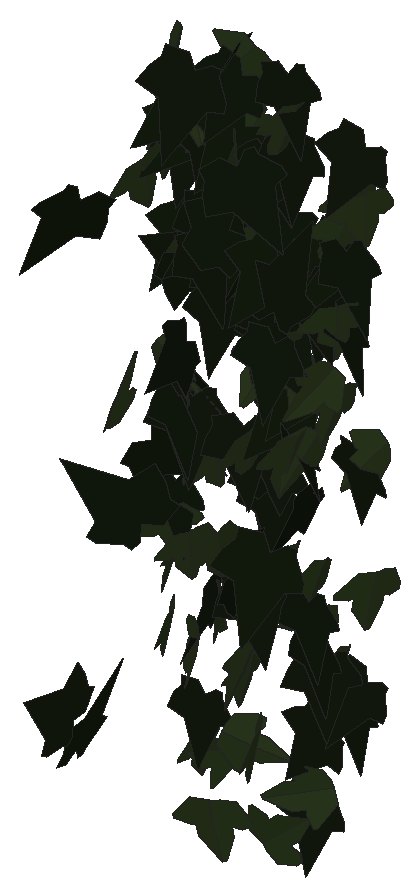
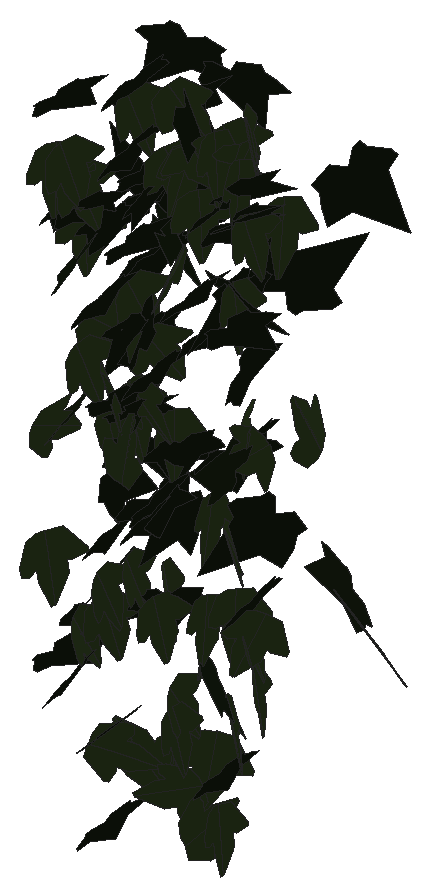
# SketchUp Ruby script. Lengths in inches.
U = 1.inch
M = Sketchup.active_model
def pt(a) = Geom::Point3d.new(a.map { |v| v * U })
def face(e, loops, mat)
  f = e.add_face(loops[0].map { |a| pt(a) })
  loops[1..].each { |l| e.add_face(l.map { |a| pt(a) }).erase! }
  f.material = f.back_material = mat if mat
  f
end
# faces: each face lists its corners as indices into pts; further lists are holes
def faces(e, pts, list, mat = nil) = list.each { |f| face(e, (f[0].is_a?(Array) ? f : [f]).map { |l| l.map { |i| pts[i] } }, mat) }
# xy, xz, yz: faces in a plane at the given z, y or x. An outline is a flat list of corners, or four numbers for a rectangle; further outlines are holes
def ring(l) = l.size == 4 ? [[l[0], l[1]], [l[2], l[1]], [l[2], l[3]], [l[0], l[3]]] : l.each_slice(2).to_a
def flat(e, list, mat, &to3) = list.each { |f| face(e, (f[0].is_a?(Array) ? f : [f]).map { |l| ring(l).map { |u, v| to3.(u, v) } }, mat) }
def xy(e, z, list, mat = nil) = flat(e, list, mat) { |x, y| [x, y, z] }
def xz(e, y, list, mat = nil) = flat(e, list, mat) { |x, z| [x, y, z] }
def yz(e, x, list, mat = nil) = flat(e, list, mat) { |y, z| [x, y, z] }
def lines(e, pts, list) = list.each { |a, b| e.add_line(pt(pts[a]), pt(pts[b])) }
# prism: a flat outline (further loops are holes) pulled along v
def prism(e, loops, v, mat = nil)
  f = face(e, loops, mat); d = Geom::Vector3d.new(v.map { |x| x * U })
  f.pushpull(f.normal.samedirection?(d) ? d.length : -d.length)
end
def box(e, o, s, mat = nil) = prism(e, [[o, [o[0] + s[0], o[1], o[2]], [o[0] + s[0], o[1] + s[1], o[2]], [o[0], o[1] + s[1], o[2]]]], [0, 0, s[2]], mat)
def at(x, y, z, deg = 0) = Geom::Transformation.translation(pt([x, y, z])) * Geom::Transformation.rotation(ORIGIN, Z_AXIS, deg.degrees)
def axes(o, x, y, z) = Geom::Transformation.new([*x, 0, *y, 0, *z, 0, *pt(o).to_a, 1])
def part(name) = M.definitions.add(name)
# library, detail: a bought-in or finely detailed component or shape, given as its bounding box
def library(name, o, s) = part(name).tap { |d| box(d.entities, o, s) }
def detail(e, o, s) = box(e.add_group.entities, o, s)
def put(e, d, t, mat = nil) = e.add_instance(d, t).tap { |i| i.material = mat if mat }
def group(e, t, mat = nil) = e.add_group.tap { |g| g.transformation = t; g.material = mat if mat }.entities
root = M.entities
M.materials.add("efeu1").color = [18, 25, 13]
M.materials.add("efeu2").color = [43, 57, 29]
c1 = part("ivyleaf_9")
p = [[1.54,2.16,1.25],[1.36,2.04,1.19],[-0.21,0.99,0.68],[-0.71,1.11,0.82],[-0.85,0.86,0.67],[-0.8,0.17,0.21],
  [-0.9,-0.01,0.1],[-0.67,-0.16,-0.02],[-0.08,-0.08,-0.05],[-0.03,-0.6,-0.4],[0.65,-0.88,-0.66],[0.83,-0.6,-0.49],
  [1.29,-0.42,-0.43],[1.8125,-0.07,-0.26],[1.21,0.44,0.15]]
faces(c1.entities,p,[[0,1,2,3,4,5,6,7,8,9,10,11,12,13,14]],"efeu1")
c2 = part("ivyleaf_10")
p = [[0,0.5,-0.03],[-0.0625,2.02,-0.43],[-0.19,2.01,-0.46],[-0.54,1.05,-0.29],[-0.52,0.625,-0.18],[-0.83,0.76,-0.28],
  [-1.16,0.64,-0.33],[-1.15,0.33,-0.24],[-0.77,-0.39,0.02],[-0.3,-0.51,0.16],[0.04,-0.48,0.23],[-0.02,2.01,-0.4375],
  [-0.06,2.01,-0.43],[0.04,-0.49,0.23],[0.67,-0.49,0.14],[1.38,0.36,-0.2],[1.375,0.51,-0.24],[0.81,0.65,-0.19],
  [0.62,0.59,-0.15],[0.6,1.09,-0.28],[0.5,1.23,-0.31]]
faces(c2.entities,p,[[0,1,2,3,4,5,6,7,8,9,10],[11,12,0,13,14,15,16,17,18,19,20]],"efeu2")
put(root,c1,axes([543.49,116.36,261.25],[0.16021,0.13331,1.3584],[-1.36181,-0.07688,0.16816],[0.0923,-1.36566,0.12313]))
put(root,c1,axes([539.99,117.03,249.64],[-0.79435,1.04419,-0.28104],[-0.1795,0.21655,1.31195],[1.06635,0.8143,0.01149]))
put(root,c1,axes([538.28,118.64,249.51],[-0.68634,0.81521,0.76926],[-0.53972,0.5502,-1.06461],[-0.98237,-0.87185,0.04745]))
put(root,c1,axes([536.61,121.2,270.97],[-0.0962,0.58477,-1.146],[0.09794,-1.14254,-0.59122],[-1.28284,-0.13108,0.0408]))
put(root,c2,axes([545.42,121.33,250.04],[0.48425,-1.06011,-0.21104],[-0.05067,0.20873,-1.16479],[1.07972,0.48525,0.03998]))
put(root,c1,axes([543.87,122.2,274.54],[-0.28215,-0.65621,-1.04476],[0.69961,0.79766,-0.68994],[1.01621,-0.73135,0.18491]))
put(root,c1,axes([544.65,123.08,257.12],[-0.95258,-0.80439,-0.37029],[0.28823,0.2326,-1.24675],[0.83731,-0.9952,0.0079]))
put(root,c1,axes([541.2,123.29,269.69],[0.21071,-1.07809,-0.24271],[0.00329,0.2477,-1.09737],[1.10507,0.20483,0.04955]))
put(root,c2,axes([541.83,123.125,244.67],[-1.16417,-0.48141,-0.08027],[0.07348,0.03237,-1.25978],[0.4825,-1.16649,-0.00183]))
put(root,c1,axes([544.15,124.03,265.95],[-0.16223,-1.09652,0.09856],[-0.00097,-0.09948,-1.10837],[1.10094,-0.16166,0.01355]))
put(root,c1,axes([541.52,124.36,270.07],[-0.54084,-0.75527,0.7338],[-0.4276,-0.59635,-0.92895],[0.96232,-0.68946,-0.00036]))
put(root,c1,axes([544.65,123.47,268.11],[-0.93397,0.54075,0.74765],[0.64265,-0.38215,1.07919],[0.66212,1.13368,0.00716]))
put(root,c1,axes([543.61,124.78,269.13],[-0.59732,-0.89897,0.39954],[-0.07958,-0.42173,-1.06789],[0.98053,-0.58187,0.15671]))
put(root,c2,axes([536.41,123.75,260.32],[0.46515,-1.08626,0.44322],[-0.17806,0.4059,1.18165],[-1.15961,-0.49805,-0.00366]))
put(root,c1,axes([540.625,124.59,270.63],[0.00315,-1.149,-0.06359],[-0.00247,0.06358,-1.149],[1.15075,0.00328,-0.0023]))
put(root,c2,axes([543.86,124.2,243.58],[-0.78365,-0.22161,0.85578],[0.82075,0.24244,0.81436],[-0.32839,1.13477,-0.00685]))
put(root,c1,axes([538.49,125.47,263.4375],[0.18138,-0.41129,-1.06261],[0.70587,-0.8041,0.43172],[-0.89445,-0.71797,0.12521]))
put(root,c1,axes([539.26,125.07,275.98],[-1.02569,-0.68214,-0.36904],[0.28672,0.23503,-1.2313],[0.72062,-1.06442,-0.03537]))
put(root,c1,axes([542.69,123.64,255.58],[-0.06573,0.22427,-1.26075],[-0.76981,1.00191,0.21836],[1.02332,0.76811,0.08329]))
put(root,c1,axes([544.99,125.22,254.07],[0.17503,-1.07468,0.03545],[0.00941,-0.03439,-1.08884],[1.07523,0.17524,0.00376]))
put(root,c1,axes([542.89,125.27,266.83],[0.00126,-1.11665,-0.03964],[0.00722,0.03965,-1.11663],[1.11733,0.001,0.00726]))
put(root,c1,axes([544.92,125.64,252.12],[0.2811,-1.02226,0.22096],[0.07578,-0.20829,-1.06006],[1.04312,0.29061,0.01747]))
put(root,c2,axes([546.17,125.44,267.41],[-0.5845,-0.96213,-0.024],[0.01113,0.02132,-1.12576],[0.96237,-0.5846,-0.00156]))
put(root,c2,axes([536.57,125.26,270.84],[-0.20419,-1.14307,-0.35777],[0.06189,0.35238,-1.16117],[1.19615,-0.21336,-0.001]))
put(root,c1,axes([537.9,125.93,260.53],[0.19278,-1.09365,0.0702],[0.01105,-0.06933,-1.11051],[1.09584,0.1931,-0.00115]))
put(root,c1,axes([544.65,125.55,268.25],[0.08852,-1.01238,-0.52262],[-0.04161,0.52097,-1.01624],[1.13856,0.09775,0.0035]))
put(root,c2,axes([543.6,125.93,260.47],[-0.09319,-1.22064,0.12956],[-0.01952,-0.12845,-1.22416],[1.22735,-0.09472,-0.00963]))
put(root,c2,axes([544.92,126.3,263.75],[0.27671,0.65594,-0.85393],[-0.55334,-0.66974,-0.69376],[-0.92373,0.59768,0.15978]))
put(root,c2,axes([542.22,126.36,263.71],[-0.65926,-0.60403,0.65453],[-0.14995,-0.72743,-0.82234],[0.87794,-0.57782,0.35104]))
put(root,c1,axes([541.96,126.02,268.82],[-0.85893,0.55562,-0.45715],[0.366,-0.27552,-1.02254],[-0.61947,-0.93319,0.02972]))
put(root,c2,axes([541.52,125.74,260.07],[-0.14878,-1.07995,-0.24936],[0.03645,0.2467,-1.09015],[1.10777,-0.15316,0.00238]))
put(root,c1,axes([539.55,126.54,265.17],[-0.08332,-1.07629,0.25389],[-0.03926,-0.25157,-1.07934],[1.10513,-0.09009,-0.01921]))
put(root,c1,axes([544.99,126.22,251.02],[-0.3834,-0.91126,-0.40207],[0.14238,0.37626,-0.98853],[0.98579,-0.40876,-0.0136]))
put(root,c1,axes([538.17,126.41,260.36],[-0.29963,-1.1328,-0.24164],[0.07424,0.2303,-1.17169],[1.15591,-0.30844,0.01261]))
put(root,c2,axes([544.59,126.28,245.17],[0.33861,0.08867,-1.07915],[-1.05405,-0.23175,-0.34978],[-0.24778,1.10703,0.01321]))
put(root,c2,axes([543,126.44,265.64],[-0.18173,-0.97374,0.46335],[0.02098,-0.47299,-0.98577],[1.07816,-0.15493,0.09728]))
put(root,c1,axes([540.33,126.83,273.18],[-0.64663,-0.87397,0.31345],[-0.17843,-0.25789,-1.08713],[0.91117,-0.67073,0.00956]))
put(root,c2,axes([540.63,125.875,272.58],[0.45892,-0.922,-0.44073],[0.04488,0.50084,-1.00103],[1.02093,0.39243,0.24211]))
put(root,c2,axes([537.22,126.13,250.5],[0.42848,-0.938,-0.19948],[-0.0357,0.20274,-1.02998],[0.95831,0.42695,0.05082]))
put(root,c1,axes([543.71,126.9,257.74],[-0.39794,0.01975,-1.03994],[0.68737,-0.83067,-0.2788],[-0.78064,-0.7415,0.28464]))
put(root,c1,axes([538.23,125.57,267.36],[0.43097,-0.44761,-1.03942],[-0.39679,0.98187,-0.58734],[1.05986,0.5496,0.20277]))
put(root,c1,axes([540.64,126.52,259.87],[-0.2609,-0.99125,-0.37424],[0.12479,0.35399,-1.02461],[1.05217,-0.28778,0.02873]))
put(root,c2,axes([543.75,126.79,260.24],[-0.15695,-0.89912,0.64092],[-0.01283,-0.64583,-0.90916],[1.1041,-0.13532,0.08054]))
put(root,c1,axes([540.03,127.08,275.24],[-0.40902,-0.97551,0.44923],[-0.07526,-0.45349,-1.05328],[1.07134,-0.40429,0.09752]))
put(root,c1,axes([542.52,126.82,263.68],[0.12712,-0.40458,1.03959],[0.5475,-0.889,-0.41292],[0.97194,0.55369,0.09664]))
put(root,c2,axes([539.86,125.9375,252.07],[0.47704,-0.75654,-0.5686],[-0.02842,0.62501,-0.85544],[0.94596,0.40029,0.26104]))
put(root,c1,axes([541.27,126.5,252.96],[-0.36466,-0.88392,-0.53568],[0.21502,0.49074,-0.95613],[1.01095,-0.42321,0.01013]))
put(root,c1,axes([545.47,126.79,266.38],[0.44387,-0.99292,0.21512],[0.06579,-0.20617,-1.08736],[1.01382,0.44809,-0.02362]))
put(root,c1,axes([538.57,126.1,266.86],[-0.58124,0.53675,0.84229],[-0.73511,0.42982,-0.78119],[-0.67614,-0.92873,0.12525]))
put(root,c1,axes([545.62,126.84,269.31],[0.27352,-1.10581,-0.19013],[-0.04012,0.18593,-1.13912],[1.12132,0.27639,0.00562]))
put(root,c1,axes([542.42,126.51,264.56],[0.09679,-0.82078,-0.76965],[0.04366,0.77465,-0.82062],[1.12434,0.04057,0.09812]))
put(root,c1,axes([538.12,127.23,246.64],[-0.05624,-1.02992,0.14554],[0.0118,-0.14638,-1.03127],[1.04009,-0.05403,0.01957]))
put(root,c2,axes([537.89,127.02,274.4],[-0.63656,-0.83611,0.45098],[-0.12717,-0.46298,-1.03786],[0.94143,-0.62789,0.16474]))
put(root,c1,axes([542.42,127.52,261.19],[-0.72708,-0.74656,0.38538],[-0.07117,-0.45309,-1.01201],[0.83714,-0.68693,0.24867]))
put(root,c1,axes([541.71,127.51,271.91],[-0.48024,-0.96745,0.34109],[-0.0575,-0.35064,-1.07548],[1.0242,-0.47331,0.09956]))
put(root,c1,axes([544.83,127.46,269.16],[-0.53214,-0.94889,0.25723],[-0.07043,-0.25495,-1.08618],[0.98061,-0.53324,0.06158]))
put(root,c2,axes([537.86,126.65,253.93],[-0.45424,-0.97776,-0.16181],[0.03991,0.15981,-1.07768],[0.99026,-0.45495,-0.03079]))
put(root,c2,axes([540.18,127.25,249.24],[0.24331,-0.95253,0.5263],[0.15331,-0.50391,-0.98289],[1.07741,0.28681,0.02101]))
put(root,c2,axes([542.55,127.1,274.37],[-0.0406,-1.10928,0.31414],[-0.00464,-0.31417,-1.11],[1.15289,-0.04033,0.00659]))
put(root,c1,axes([542.72,127.27,259.86],[0.44716,-0.83404,0.51296],[0.25347,-0.4461,-0.94628],[0.94578,0.51389,0.01108]))
put(root,c2,axes([537.95,126.1,261.01],[-0.29549,0.55739,-1.02446],[-0.52848,0.87811,0.63019],[1.03967,0.60478,0.02917]))
put(root,c2,axes([537.72,126.79,267.46],[-0.03502,-1.08991,-0.11285],[0.02146,0.11221,-1.09032],[1.09552,-0.03704,0.01775]))
put(root,c1,axes([545.78,127.59,273.78],[-0.48887,-0.96241,0.31879],[-0.05341,-0.32897,-1.07507],[1.01242,-0.48207,0.09722]))
put(root,c2,axes([536.8,127.16,253.22],[0.45481,-0.96083,0.18533],[0.05187,-0.18041,-1.06262],[0.97716,0.45679,-0.02985]))
put(root,c2,axes([544.88,127.34,250.73],[0.29188,-0.92671,0.45216],[0.13221,-0.43242,-0.97158],[1.02262,0.32041,-0.00345]))
put(root,c2,axes([544.83,127.27,262.53],[-0.08776,-1.04924,0.33224],[0.02369,-0.33502,-1.05175],[1.10033,-0.07647,0.04914]))
put(root,c1,axes([536.47,126.1875,258.02],[0.02571,-0.09389,-1.23097],[0.02704,1.23098,-0.09333],[1.23425,-0.02501,0.02769]))
put(root,c2,axes([545.01,127.36,270.25],[-0.2963,-1.01829,0.39619],[-0.02953,-0.40289,-1.05759],[1.09225,-0.28713,0.07888]))
put(root,c1,axes([543.56,127.9,246.65],[-0.43178,-0.78665,0.66719],[0.0204,-0.72966,-0.84711],[1.03129,-0.31493,0.2961]))
put(root,c1,axes([541.28,127.56,256.99],[0.04924,-1.09588,0.10407],[0.02687,-0.10294,-1.09677],[1.10048,0.05155,0.02212]))
put(root,c1,axes([536.98,127.89,272.78],[-0.70377,-0.678,0.57243],[-0.26396,-0.53758,-0.96124],[0.84716,-0.73074,0.17604]))
put(root,c2,axes([541.24,127.23,252.68],[-0.25724,-1.02638,0.14823],[0.01052,-0.1553,-1.05706],[1.03698,-0.25304,0.0475]))
put(root,c2,axes([537.94,126.75,249.26],[0.55172,-0.79291,-0.71078],[-0.3796,0.60148,-0.96563],[0.99489,0.6692,0.02573]))
put(root,c1,axes([545.74,127.79,249.625],[-0.50159,-0.87184,0.30464],[-0.13696,-0.27262,-1.00569],[0.91332,-0.51969,0.01649]))
put(root,c1,axes([539.32,127.86,267.25],[-0.22479,-1.03025,0.37247],[0.03298,-0.38642,-1.04893],[1.09501,-0.19986,0.10806]))
put(root,c1,axes([536.81,127.99,271.5],[-0.68916,-0.75384,0.48854],[-0.05173,-0.58142,-0.97013],[0.89681,-0.61283,0.31947]))
put(root,c2,axes([537.59,126.94,273.86],[0.34888,1.06413,0.14299],[0.06263,0.12992,-1.1197],[-1.07187,0.35395,-0.01888]))
put(root,c1,axes([542.29,127.72,272.7],[0.0301,-1.13304,0.14401],[-0.00733,-0.14425,-1.13339],[1.14213,0.02893,-0.01107]))
put(root,c1,axes([545.52,127.82,259.53],[0.09969,-0.9481,0.51024],[0.17731,-0.49097,-0.94694],[1.06198,0.17097,0.1102]))
put(root,c1,axes([542.09,127.52,275.76],[0.16039,-1.10682,-0.1239],[-0.01239,0.1234,-1.11837],[1.11367,0.16078,0.0054]))
put(root,c2,axes([536.22,127.3125,261.54],[-0.71961,0.13681,-0.83108],[0.76739,-0.34405,-0.7211],[-0.34716,-1.04411,0.12872]))
put(root,c1,axes([537.95,127.9,271.63],[-0.08721,-1.08107,0.25852],[0.02645,-0.26126,-1.0836],[1.11123,-0.07862,0.04608]))
put(root,c2,axes([536.57,127.41,275.58],[0.67556,-0.89557,0.08296],[0.12858,-0.00652,-1.11747],[0.89016,0.68061,0.09845]))
put(root,c2,axes([542.12,127.59,254.29],[0.28247,-1.005,0.27621],[0.07515,-0.26579,-1.04394],[1.03955,0.2923,0.00041]))
put(root,c2,axes([538.66,127.08,257.98],[0.00213,-1.00701,-0.39543],[0.11128,0.39354,-1.00159],[1.07613,-0.0387,0.10436]))
put(root,c2,axes([543.49,127.55,252.07],[-0.39794,-0.95193,0.27209],[-0.03624,-0.27905,-1.02926],[0.98939,-0.3931,0.07174]))
put(root,c2,axes([538.7,128.13,244.14],[-0.15455,-0.27137,-1.10559],[-0.42077,-1.0231,0.30995],[-1.05779,0.44662,0.03824]))
put(root,c1,axes([545.04,127.76,248.71],[0.24827,-1.02616,0.13462],[0.02836,-0.13165,-1.05576],[1.03456,0.24986,-0.00337]))
put(root,c1,axes([536.99,127.98,271.49],[-0.30016,-1.07769,0.07527],[-0.01135,-0.07497,-1.11867],[1.08026,-0.30023,0.00916]))
put(root,c2,axes([540.24,127.72,272.94],[-0.6361,-0.8307,0.41785],[-0.148,-0.40937,-1.03913],[0.91802,-0.64159,0.12201]))
put(root,c2,axes([537.14,127.26,273.17],[0.0185,-1.07942,-0.36029],[0.06974,0.36074,-1.07717],[1.13582,-0.00457,0.072]))
put(root,c1,axes([541.1,127.86,257.82],[-0.37022,-0.98904,-0.18845],[0.04611,0.18392,-1.05585],[1.00577,-0.3725,-0.02096]))
put(root,c2,axes([539.71,127.25,245.46],[-0.3532,-0.13813,-1.03534],[1.03302,0.11553,-0.36782],[0.15456,-1.08781,0.09241]))
put(root,c2,axes([536.38,127.75,271.36],[-0.02482,-1.09835,0.21788],[0.01546,-0.21825,-1.09845],[1.11965,-0.02133,0.02]))
put(root,c2,axes([537.93,127.46,244.82],[-0.0053,-1.04896,-0.16508],[0.02448,0.16491,-1.04871],[1.06159,-0.00904,0.02335]))
put(root,c1,axes([538.36,127.75,251.31],[-0.92587,0.45968,-0.57096],[0.5188,-0.23886,-1.0336],[-0.51783,-1.06121,-0.01468]))
put(root,c2,axes([545.22,127.82,271.39],[-0.2414,-1.07051,0.30346],[-0.00055,-0.31041,-1.09545],[1.11269,-0.2324,0.0653]))
put(root,c1,axes([536.08,127.97,255.2],[0.17602,-1.06453,0.05599],[0.01581,-0.05413,-1.07896],[1.06588,0.1766,0.00676]))
put(root,c1,axes([536.875,128.23,267.05],[-0.65613,-0.85463,0.24147],[-0.16715,-0.17602,-1.07716],[0.87221,-0.67663,-0.02478]))
put(root,c1,axes([541.73,128.39,269.15],[-0.44445,-0.91237,0.45193],[-0.13484,-0.43602,-1.01287],[1.0092,-0.46007,0.0637]))
put(root,c2,axes([541.875,127.48,262.15],[0.69427,-0.37417,-0.80668],[-0.72593,0.35259,-0.78832],[0.51357,1.0042,-0.02378]))
put(root,c1,axes([537,127.86,260.6],[0.6769,-0.73553,0.41424],[0.34858,-0.24005,-0.99582],[0.76883,0.75641,0.08679]))
put(root,c1,axes([539.14,128.01,275.68],[-0.6142,0.4812,-0.81978],[0.56168,-0.60368,-0.77518],[-0.76688,-0.82755,0.0888]))
put(root,c2,axes([538.58,127.48,253.77],[-0.13661,-1.01579,-0.30349],[0.07427,0.29608,-1.02442],[1.05756,-0.15201,0.03274]))
put(root,c1,axes([542.57,128.39,261.99],[-0.6527,-0.80833,0.30515],[-0.09099,-0.316,-1.0317],[0.8592,-0.64752,0.12255]))
put(root,c2,axes([539.51,127.46,273.15],[-0.43085,-0.9586,-0.40807],[0.28149,0.31806,-1.04436],[1.0031,-0.50099,0.11779]))
put(root,c1,axes([542.9,128.29,243.28],[-0.10122,-1.0861,0.17831],[0.00255,-0.17929,-1.09064],[1.10064,-0.09946,0.01893]))
put(root,c2,axes([539.79,127.91,275.9],[-0.77306,-0.28997,0.77562],[-0.66312,-0.4187,-0.81746],[0.49592,-1.01187,0.11599]))
put(root,c2,axes([536.08,127.48,253.9],[-0.82289,-0.52091,-0.42514],[0.34806,0.24487,-0.97372],[0.57528,-0.89327,-0.019]))
put(root,c1,axes([540.51,128.49,258.22],[-0.20153,-0.96439,0.4365],[-0.06573,-0.43208,-0.98498],[1.05654,-0.21083,0.02198]))
put(root,c2,axes([545.7,128.55,259.76],[-0.25831,-0.3332,1.00297],[0.15718,-1.03312,-0.30273],[1.04512,0.07303,0.29343]))
put(root,c2,axes([537.93,127.73,274.35],[-0.11123,-1.11497,-0.16054],[0.02031,0.1593,-1.12049],[1.12628,-0.11299,0.00435]))
put(root,c2,axes([539.83,127.91,248.57],[0.06859,-1.06761,0.04154],[-0.00359,-0.04186,-1.06979],[1.06841,0.0684,-0.00626]))
put(root,c1,axes([543.12,128.37,266.17],[0.00976,-1.10197,0.19045],[0.00439,-0.19042,-1.10201],[1.1183,0.01036,0.00266]))
put(root,c2,axes([541.98,128.46,259.19],[-0.07801,-0.79421,-0.75869],[0.07134,-0.76265,0.79103],[-1.09603,0.00689,0.10548]))
put(root,c2,axes([543.06,128.2,253.61],[0.14115,-1.00933,0.37026],[0.10373,-0.35891,-1.01793],[1.07008,0.16793,0.04984]))
put(root,c2,axes([545.67,127.85,271.22],[-0.51543,-1.00778,-0.09552],[0.04918,0.08214,-1.13192],[1.0111,-0.51773,0.00636]))
put(root,c2,axes([540.06,127.3125,268.48],[0.48616,-0.72671,-0.71756],[0.23844,0.85352,-0.70286],[0.99305,0.15084,0.52005]))
put(root,c1,axes([540.52,128.49,263.91],[-0.02122,-1.08647,0.13075],[0.01545,-0.13106,-1.08653],[1.0942,-0.01922,0.01787]))
put(root,c2,axes([538.61,128.16,274.17],[0.66217,0.8138,-0.41376],[-0.25009,-0.32989,-1.04908],[-0.87802,0.7077,-0.01323]))
put(root,c2,axes([536.9,128.19,257.71],[0.74064,-0.75181,0.17822],[0.11754,-0.13437,-1.05531],[0.76366,0.74984,-0.01042]))
put(root,c1,axes([540.6,128.13,271.86],[0.31526,-1.03402,-0.27569],[-0.07769,0.26453,-1.08101],[1.06732,0.32468,0.00275]))
put(root,c2,axes([545.9375,128.06,254.22],[-0.46499,-1.06092,0.0823],[-0.01524,-0.08316,-1.15818],[1.064,-0.46483,0.01938]))
put(root,c2,axes([542.98,128.08,262.39],[0.80956,-0.74256,-0.07024],[-0.05206,0.04716,-1.09854],[0.74406,0.81123,-0.00044]))
put(root,c2,axes([538.54,128.01,271.72],[-0.549,-0.9803,0.01438],[0.01254,-0.0235,-1.12333],[0.98032,-0.54868,0.02243]))
